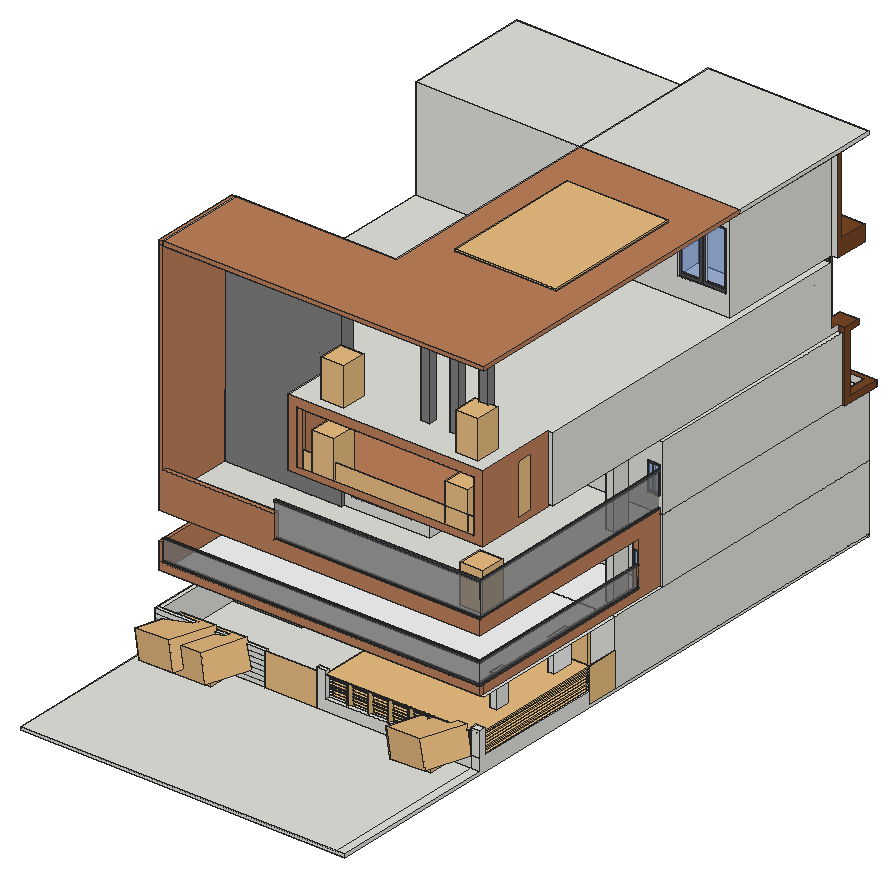
# SketchUp Ruby script. Lengths in inches.
U = 1.inch
M = Sketchup.active_model
def pt(a) = Geom::Point3d.new(a.map { |v| v * U })
def face(e, loops, mat)
  f = e.add_face(loops[0].map { |a| pt(a) })
  loops[1..].each { |l| e.add_face(l.map { |a| pt(a) }).erase! }
  f.material = f.back_material = mat if mat
  f
end
# faces: each face lists its corners as indices into pts; further lists are holes
def faces(e, pts, list, mat = nil) = list.each { |f| face(e, (f[0].is_a?(Array) ? f : [f]).map { |l| l.map { |i| pts[i] } }, mat) }
# xy, xz, yz: faces in a plane at the given z, y or x. An outline is a flat list of corners, or four numbers for a rectangle; further outlines are holes
def ring(l) = l.size == 4 ? [[l[0], l[1]], [l[2], l[1]], [l[2], l[3]], [l[0], l[3]]] : l.each_slice(2).to_a
def flat(e, list, mat, &to3) = list.each { |f| face(e, (f[0].is_a?(Array) ? f : [f]).map { |l| ring(l).map { |u, v| to3.(u, v) } }, mat) }
def xy(e, z, list, mat = nil) = flat(e, list, mat) { |x, y| [x, y, z] }
def xz(e, y, list, mat = nil) = flat(e, list, mat) { |x, z| [x, y, z] }
def yz(e, x, list, mat = nil) = flat(e, list, mat) { |y, z| [x, y, z] }
def lines(e, pts, list) = list.each { |a, b| e.add_line(pt(pts[a]), pt(pts[b])) }
# prism: a flat outline (further loops are holes) pulled along v
def prism(e, loops, v, mat = nil)
  f = face(e, loops, mat); d = Geom::Vector3d.new(v.map { |x| x * U })
  f.pushpull(f.normal.samedirection?(d) ? d.length : -d.length)
end
def box(e, o, s, mat = nil) = prism(e, [[o, [o[0] + s[0], o[1], o[2]], [o[0] + s[0], o[1] + s[1], o[2]], [o[0], o[1] + s[1], o[2]]]], [0, 0, s[2]], mat)
def at(x, y, z, deg = 0) = Geom::Transformation.translation(pt([x, y, z])) * Geom::Transformation.rotation(ORIGIN, Z_AXIS, deg.degrees)
def axes(o, x, y, z) = Geom::Transformation.new([*x, 0, *y, 0, *z, 0, *pt(o).to_a, 1])
def part(name) = M.definitions.add(name)
# library, detail: a bought-in or finely detailed component or shape, given as its bounding box
def library(name, o, s) = part(name).tap { |d| box(d.entities, o, s) }
def detail(e, o, s) = box(e.add_group.entities, o, s)
def put(e, d, t, mat = nil) = e.add_instance(d, t).tap { |i| i.material = mat if mat }
def group(e, t, mat = nil) = e.add_group.tap { |g| g.transformation = t; g.material = mat if mat }.entities
root = M.entities
M.materials.add("GATE RAILINGS").color = [40, 40, 40]
M.materials.add("Material__1").color = [190, 136, 85]
M.materials.add("Material__2").color = [51, 42, 44]
M.materials.add("Material__3").color = [119, 136, 107]
M.materials.add("[0129_WhiteSmoke]").color = [245, 245, 245]
M.materials.add("[0133_Gray]").color = [128, 128, 128]
M.materials.add("[0134_DimGray]").color = [105, 105, 105]
M.materials.add("[0135_DarkGray]").color = [81, 81, 81]
M.materials.add("[Aluminum]1").color = [79, 79, 79]
M.materials.add("[Color_000]").color = [255, 255, 255]
M.materials.add("[Translucent Glass Blue]").color = [100, 149, 237]
M.materials["[Translucent Glass Blue]"].alpha = 0.5
M.materials.add("[Translucent Glass Gray]").color = [128, 128, 128]
M.materials["[Translucent Glass Gray]"].alpha = 0.5
M.materials.add("[Wood Veneer 01]1").color = [120, 70, 37]
M.materials.add("[Wood Veneer 02]").color = [190, 128, 91]
c1 = library("jali15",[0,0,0],[42.92,2.71,85.83])
c2 = library("e203.dxf",[0,0,0],[1.18,1.18,0.01])
c3 = part("Janela aluminio")
xy(c3.entities,0,[[0,0,47.24,1.57],[23.62,1.57,47.24,2.76],[0,2.76,25.98,3.9375],[0,3.9375,47.24,5.91]])
xy(c3.entities,43.31,[[0,0,47.24,1.57],[23.62,1.57,47.24,2.76],[0,2.76,0,5.91,47.24,5.91,47.24,3.9375,25.98,3.9375,25.98,2.76],[25.98,2.76,47.24,3.9375]])
xz(c3.entities,1.57,[[0,0,23.62,0,23.62,41.34,21.26,41.34,21.26,1.97,1.97,1.97,1.97,41.34,23.62,41.34,23.62,43.31,0,43.31],[[23.62,0,47.24,43.31],[25.7,1.97,45.28,41.34]]],"[0135_DarkGray]")
xz(c3.entities,2.76,[[[0,0,23.62,43.31],[2.36,2.36,21.26,40.94]],[23.62,0,25.98,43.31]],"[0135_DarkGray]")
xz(c3.entities,2.76,[[2.36,2.36,21.26,40.94]],"[Translucent Glass Blue]")
xz(c3.entities,3.9375,[[25.98,0,25.98,2.36,44.88,2.36,44.88,40.94,25.98,40.94,25.98,43.31,47.24,43.31,47.24,0]],"[0135_DarkGray]")
xz(c3.entities,3.9375,[[25.98,2.36,44.88,40.94]],"[Translucent Glass Blue]")
yz(c3.entities,0,[[0,0,1.57,43.31],[2.76,0,5.91,43.31]])
yz(c3.entities,23.62,[[1.57,0,2.76,43.31]])
yz(c3.entities,25.98,[[2.76,0,3.9375,43.31]])
yz(c3.entities,47.24,[[0,0,1.57,43.31],[1.57,0,2.76,43.31],[3.9375,0,5.91,43.31]])
c4 = part("bod vindu")
g1 = group(c4.entities,at(0,-46.85,0),"[Translucent Glass Blue]")
yz(g1,0.94,[[2.36,2.36,44.49,19.65]],"[Translucent Glass Blue]")
p = [[0.55,44.49,2.36],[0.94,44.49,2.36],[0.55,2.36,19.65],[0.94,2.36,19.65]]
lines(g1,p,[[0,1],[2,3]])
g2 = group(g1,at(0,46.85,0,-90),"[Color_000]")
xy(g2,0,[[0,0,46.85,3.9375]],"[0135_DarkGray]")
xy(g2,1.57,[[1.57,0,45.28,0.55]],"[0135_DarkGray]")
xy(g2,2.36,[[2.36,0.55,44.49,3.9375]],"[0135_DarkGray]")
xy(g2,19.65,[[2.36,0.55,4.29,3.9375],[4.29,0.55,44.49,3.9375]],"[0135_DarkGray]")
xy(g2,20.43,[[1.57,0,45.28,0.55]],"[0135_DarkGray]")
xy(g2,22.01,[[0,0,46.85,3.9375]],"[0135_DarkGray]")
xz(g2,0,[[[0,0,46.85,22.01],[1.57,1.57,45.28,20.43]]],"[0135_DarkGray]")
xz(g2,0.55,[[1.57,1.57,45.28,2.36],[1.57,2.36,2.36,2.36,2.36,19.65,44.49,19.65,44.49,2.36,45.28,2.36,45.28,20.43,1.57,20.43]],"[0135_DarkGray]")
xz(g2,3.9375,[[[0,0,46.85,22.01],[2.36,2.36,44.49,19.65]]],"[0135_DarkGray]")
yz(g2,0,[[0,0,3.9375,22.01]],"[0135_DarkGray]")
yz(g2,1.57,[[0,1.57,0.55,2.36,0.55,20.43,0,20.43]],"[0135_DarkGray]")
yz(g2,2.36,[[0.55,2.36,3.9375,19.65]],"[0135_DarkGray]")
yz(g2,44.49,[[0.55,2.36,3.9375,19.65]],"[0135_DarkGray]")
yz(g2,45.28,[[0,1.57,0,20.43,0.55,20.43,0.55,2.36]],"[0135_DarkGray]")
yz(g2,46.85,[[0,0,3.9375,22.01]],"[0135_DarkGray]")
p = [[45.28,0,1.57],[1.57,0,1.57],[1.57,0.55,2.36],[2.36,0.55,2.36],[44.49,0.55,2.36],[45.28,0.55,2.36]]
faces(g2,p,[[0,1,2,3,4,5]],"[0135_DarkGray]")
c5 = part("glassesrail")
p = [[933.04,699.08,19.69],[933.04,702.23,19.69]]
lines(c5.entities,p,[[0,1]])
g3 = group(c5.entities,at(14.48,46.28,19.69))
xz(g3,0,[[0.02,0,187.07,0.79,187.06,2.76,0.01,1.97],[0.01,33.46,187.06,34.25,187.05,36.22,0,35.43]],"[Aluminum]1")
xz(g3,1.97,[[0.8,0,0.8,1.97,187.06,2.76,187.07,0.79],[1.98,33.47,1.97,35.44,187.05,36.22,187.06,34.25]],"[Aluminum]1")
p = [[0.8,1.97,0],[0.8,249.26,0],[0.02,249.26,0],[0.02,0,0],[187.07,0,0.79],[187.07,1.97,0.79],
  [0.01,0,1.97],[0.01,249.26,1.97],[0.8,1.97,1.97],[0.8,249.26,1.97],[187.06,0,2.76],[187.06,1.97,2.76],
  [0.01,249.26,33.46],[0.66,249.26,33.47],[1.06,249.26,33.47],[1.98,249.26,33.47],[1.98,1.97,33.47],[187.06,1.97,34.25],
  [187.06,0,34.25],[0.01,0,33.46],[0,0,35.43],[0,249.26,35.43],[1.97,249.26,35.44],[1.97,1.97,35.44],
  [187.05,0,36.22],[187.05,1.97,36.22]]
faces(g3,p,[[0,1,2,3,4,5],[6,7,2,3],[8,9,7,6,10,11],[12,13,14,15,16,17,18,19],[20,21,12,19],[16,15,22,23],[23,22,21,20,24,25]],"[Aluminum]1")
g4 = group(g3,at(0.8,411.86,1.97))
prism(g4,[[[0,-411.07,0],[0,-162.6,0],[0.39,-162.6,0],[0.39,-410.68,0],[185.47,-410.68,0.78],[185.47,-411.07,0.78]]],[-0.13,0,31.5],"[Translucent Glass Gray]")
c6 = library("Glass Railings(black Handrails)",[-57.04,-132.55,0],[169.29,2.52,28.17])
c7 = library("3+80",[0,-4.72,-0.01],[36.22,7.09,85.04])
c8 = library("Porton casa",[13.02,-50.57,0],[86.62,1.75,86.61])
c9 = library("Horizontal railing bar",[-171.26,0.98,-0.71],[237.2,23.72,0.71])
c10 = library("Railing post",[0,-1.77,-6.85],[2.07,1.28,39.37])
c11 = library("Group\#90",[-171.26,0,0],[238.19,24.7,1.97])
c12 = part("Balcony railing")
put(c12.entities,c9,at(44.24,-0.6875,35.43),"GATE RAILINGS")
put(c12.entities,c9,at(44.24,-0.6875,30.79),"GATE RAILINGS")
put(c12.entities,c9,at(44.24,-0.6875,26.14),"GATE RAILINGS")
put(c12.entities,c9,at(44.24,-0.6875,21.5),"GATE RAILINGS")
put(c12.entities,c9,at(44.24,-0.6875,16.85),"GATE RAILINGS")
put(c12.entities,c9,at(44.24,-0.6875,12.2),"GATE RAILINGS")
put(c12.entities,c9,at(44.24,-0.6875,7.56),"GATE RAILINGS")
put(c12.entities,c10,at(60.92,1.38,6.85))
put(c12.entities,c10,at(92.41,1.38,6.85))
put(c12.entities,c10,at(29.42,1.38,6.85))
put(c12.entities,c10,at(-2.07,1.38,6.85))
put(c12.entities,c10,at(-33.57,1.38,6.85))
put(c12.entities,c10,at(-65.07,1.38,6.85))
put(c12.entities,c10,at(-96.5625,1.38,6.85))
put(c12.entities,c11,at(44.24,-0.6875,39.37),"GATE RAILINGS")
c13 = library("Modern Gate 1",[0,0,0],[118.11,1.97,78.74])
c14 = library("cay+chuoi",[26.89,19.66,0.52],[41.96,45.65,69.71])
c15 = library("\#2",[-119.83,-119.83,113.8],[239.66,239.66,17.4])
c16 = library("\#4",[-204.92,-212.35,-236.71],[424.28,257.5,472.53])
c17 = part("\#3")
put(c17.entities,c16,axes([-0.37,309.72,0],[1.36765,0,0],[0,1.36765,0],[0,0,1.36765]),"Material__3")
c18 = library("\#1",[-174.07,-174.07,0],[348.14,348.14,140])
c19 = part("9")
put(c19.entities,c15,at(-19.94,-24.66,0),"Material__2")
put(c19.entities,c17,axes([17.67,-32.6,40.29],[0.29694,0.9549,0],[-0.21403,0.06656,0.97456],[0.9306,-0.28939,0.22414]))
put(c19.entities,c18,at(-19.94,-24.66,0),"Material__1")
xy(root,-6,[[0,0,600,1207],[0,1207,600,1207.75]])
xy(root,0,[[0,0,583.5,310.875],[583.5,0,600,310.875],[203.51,310.875,298.89,317.875],[8,317.875,583.5,317.875,583.5,566.56,600,566.56,600,621.75,324.89,621.75,324.89,484.6875,135.89,484.6875,135.89,480.875,8,480.875],[0,480.875,135.89,480.875,135.89,484.6875,324.89,484.6875,324.89,621.75,600,621.75,600,1207,0,1207],
  [0,1207,600,1207.75]])
xy(root,7.16,[[318.64,517.94,324.89,595.69]])
xy(root,9.32,[[152.3125,484.6875,291.25,502.875]])
xy(root,21.25,[[316.34,310.875,583.5,317.875],[583.5,323.28,600,566.56]])
xy(root,60,[[0,310.875,203.51,317.875],[0,317.875,8,480.875]])
xy(root,67.0625,[[298.89,310.875,316.34,317.875],[583.5,310.875,600,323.28]])
xy(root,101.2,[[152.3125,484.6875,291.25,502.875]])
xy(root,102.03,[[318.64,517.94,324.89,595.69]])
xy(root,120,[[594.25,319,600,621.75],[0,327,8,480.875],[0,480.875,8,488.375],[0,488.375,0,1207.75,600,1207.75,600,732.75,381.34,732.75,381.34,621.75,324.89,621.75,324.89,495.125,165.85,495.125,165.85,488.375],[324.89,495.125,381.34,621.75],
  [561.82,515.52,572.89,555.2],[583.49,621.75,594.25,732.75],[594.25,621.75,600,732.75],[562.02,648.71,577.08,680.89]])
xy(root,120,[[0,319,594.25,327],[[8,327,8,480.875,135.89,480.875,135.89,484.6875,324.89,484.6875,324.89,495.125,381.34,495.125,381.34,621.75,583.49,621.75,583.49,327],[561.82,515.52,572.89,555.2]],[[583.49,327,594.25,621.75],[561.82,381.16,574.2,408.78]],[8,480.875,8,488.375,165.85,488.375,165.85,495.125,324.89,495.125,324.89,484.6875,135.89,484.6875,135.89,480.875],[[381.34,621.75,583.49,732.75],[562.02,648.71,577.08,680.89]]],"[0129_WhiteSmoke]")
xy(root,127.77,[[362.03,644.59,381.34,705.65]])
xy(root,132.96,[[177.95,495.125,345.45,525.4375]])
xy(root,134.375,[[0,319,8,327]])
xy(root,134.375,[[8,319,594.25,327],[583.49,327,594.25,684.5625]],"[Wood Veneer 02]")
xy(root,168,[[0,319,8,488.375]],"[Wood Veneer 02]")
xy(root,172.76,[[585.65,684.5625,592.33,691]])
xy(root,199.19,[[585.65,684.5625,592.33,691]])
xy(root,200.65,[[362.03,644.59,381.34,705.65]])
xy(root,206.77,[[177.95,495.125,345.45,525.4375]])
xy(root,218.53,[[0,319,0,488.375,31.26,488.375,31.26,354.9375,583.49,354.9375,583.49,684.5625,594.25,684.5625,594.25,319],[31.26,354.9375,31.26,488.375,165.85,488.375,165.85,495.125,381.34,495.125,381.34,732.75,583.49,732.75,583.49,354.9375]],"[Wood Veneer 02]")
xy(root,240,[[8,327,586.25,327,586.25,732.75,381.34,732.75,381.34,468.0625,223.57,468.0625,223.57,462,8,462],[8,462,8,488.375,0,488.375,0,1145.375,600,1145.375,600,732.75,381.34,732.75,381.34,468.0625,223.57,468.0625,223.57,462],[[0,1145.375,591.125,1207.75],[535.76,1182.9375,537.8,1183.37,539.66,1184.32,541.22,1185.72,542.36,1187.47,543,1189.45,543.11,1191.54,542.68,1193.58,541.73,1195.44,540.33,1197,538.58,1198.13,536.6,1198.78,534.51,1198.89,532.47,1198.46,530.61,1197.51,529.06,1196.11,527.92,1194.36,527.27,1192.375,527.16,1190.29,527.59,1188.25,528.54,1186.39,529.9375,1184.83,531.6875,1183.7,533.67,1183.05]],[591.125,1145.375,600,1207.75],[600,1145.375,606.25,1218.25],
  [535.76,1182.9375,533.67,1183.05,531.6875,1183.7,529.9375,1184.83,528.54,1186.39,527.59,1188.25,527.16,1190.29,527.27,1192.375,527.92,1194.36,529.06,1196.11,530.61,1197.51,532.47,1198.46,534.51,1198.89,536.6,1198.78,538.58,1198.13,540.33,1197,541.73,1195.44,542.68,1193.58,543.11,1191.54,543,1189.45,542.36,1187.47,541.22,1185.72,539.66,1184.32,537.8,1183.37],[0,1207.75,600,1218.25]])
xy(root,245.125,[[214.63,319,594.25,319,594.25,732.75,586.25,732.75,586.25,327,214.63,327]],"[Wood Veneer 02]")
xy(root,252.33,[[591.125,1157.8125,606.25,1157.8125,606.25,1218.25,0,1218.25,0,1207.75,591.125,1207.75]],"[Wood Veneer 01]1")
xy(root,257.15,[[366.9,548.34,381.34,682.41]])
xy(root,258.5625,[[238.35,468.0625,348.91,499.75]])
xy(root,269.16,[[572.59,732.75,593.96,740.9375]])
xy(root,288,[[8,319,214.63,327]],"[Wood Veneer 02]")
xy(root,321.6,[[572.59,732.75,593.96,740.9375]])
xy(root,332.02,[[366.9,548.34,381.34,682.41]])
xy(root,335,[[238.35,468.0625,348.91,499.75]])
xy(root,354.5625,[[223.57,468.0625,381.34,487.75]])
xy(root,354.5625,[[223.57,337.625,223.57,468.0625,381.34,468.0625,381.34,487.75,584.16,487.75,584.16,337.625]],"[Wood Veneer 02]")
xy(root,360,[[0,462,8,488.375],[[381.34,487.75,592.625,732.75],[562.02,648.71,577.08,680.89]],[592.625,732.75,600,1145.375],[0,1091.625,584.625,1145.375],[584.625,1091.625,592.625,1145.375]])
xy(root,360,[[571.27,1145.375,571.27,1177.4375,606.25,1177.4375,606.25,1157.8125,591.125,1157.8125,591.125,1145.375]],"[Wood Veneer 01]1")
xy(root,366,[[240.32,337.625,251.32,341.6875]])
xy(root,366,[[251.32,337.625,567.35,337.625,567.35,487.75,240.32,487.75,240.32,341.6875,251.32,341.6875]],"[Wood Veneer 02]")
xy(root,368.23,[[581.85,419.93,584.16,446.93]])
xy(root,370.12,[[578.4375,1091.625,584.625,1130]])
xy(root,370.12,[[0,1091.625,578.4375,1091.625,578.4375,1130,592.625,1130,592.625,1145.375,606.25,1145.375,606.25,1177.4375,571.27,1177.4375,571.27,1145.375,0,1145.375]],"[Wood Veneer 01]1")
xy(root,372.74,[[290.9,487.75,461.27,551.125]])
xy(root,455.86,[[290.9,487.75,461.27,551.125]])
xy(root,458.42,[[581.85,419.93,584.16,446.93]],"[Wood Veneer 02]")
xy(root,464.6875,[[251.32,337.625,251.32,341.6875,240.32,341.6875,240.32,487.75,567.35,487.75,567.35,337.625]],"[Wood Veneer 02]")
xy(root,480,[[[223.57,337.625,584.16,337.625,584.16,487.75,592.625,487.75,592.625,1130,580.6875,1130,580.6875,911.92,0,911.92,0,487.75,223.57,487.75],[420.56,398.17,437.44,411.49],[474.66,398.17,491.53,411.49],[528.75,398.17,545.63,411.49]],[[0,1091.625,0,1207.75,592.625,1207.75,592.625,1145.375,578.4375,1145.375,578.4375,1091.625],[535.76,1182.9375,537.8,1183.37,539.66,1184.32,541.22,1185.72,542.36,1187.47,543,1189.45,543.11,1191.54,542.68,1193.58,541.73,1195.44,540.33,1197,538.58,1198.13,536.6,1198.78,534.51,1198.89,532.47,1198.46,530.61,1197.51,529.06,1196.11,527.92,1194.36,527.27,1192.375,527.16,1190.29,527.59,1188.25,528.54,1186.39,529.9375,1184.83,531.6875,1183.7,533.67,1183.05]],[578.4375,1130,580.6875,1145.375]])
xy(root,509.8125,[[0,1145.375,573,1145.375,573,1153.6875,592.625,1153.6875,592.625,1207.75,0,1207.75]],"[Wood Veneer 01]1")
xy(root,516.3125,[[484.875,911.92,572.5,958.23]])
xy(root,625.25,[[484.875,911.92,572.5,958.23]])
xy(root,651.0625,[[528.75,398.17,545.63,411.49]])
xy(root,658.8125,[[0,319,8,462],[8,462,223.57,487.75],[580.6875,911.92,600,1145.375],[304,1145.375,573,1207.75],[592.625,1145.375,600,1207.75],
  [573,1153.6875,592.625,1207.75]])
xy(root,658.8125,[[[8,319,8,462,223.57,462,223.57,487.75,304,487.75,304,1145.375,580.6875,1145.375,580.6875,911.92,600,911.92,600,319],[355.23,559.36,541.86,818.43],[420.56,398.17,437.44,411.49],[474.66,398.17,491.53,411.49]]],"[Wood Veneer 02]")
xy(root,665.9375,[[0,911.92,304,1145.375],[304,911.92,600,1207.75]])
xy(root,665.9375,[[0,319,8,488.375],[[8,319,600,319,600,911.92,304,911.92,304,487.75,8,487.75],[355.23,559.36,541.86,818.43]]],"[Wood Veneer 02]")
xz(root,0,[[0,-6,600,0]])
xz(root,310.875,[[0,0,203.51,60],[298.89,0,583.5,0,583.5,21.25,316.34,21.25,316.34,67.0625,298.89,67.0625],[583.5,0,600,21.25],[583.5,21.25,600,67.0625]])
xz(root,317.875,[[8,0,203.51,60],[298.89,0,298.89,67.0625,316.34,67.0625,316.34,21.25,583.5,21.25,583.5,0]])
xz(root,319,[[0,120,594.25,134.375],[0,134.375,8,168],[0,218.53,594.25,218.53,594.25,245.125,214.63,245.125,214.63,288,8,288,8,658.8125,0,658.8125],[0,658.8125,8,665.9375],[8,658.8125,600,665.9375]],"[Wood Veneer 02]")
xz(root,323.28,[[583.5,21.25,600,67.0625]])
xz(root,327,[[0,120,8,134.375],[583.49,120,594.25,134.375]])
xz(root,327,[[8,120,583.49,134.375],[8,240,214.63,288],[214.63,240,586.25,245.125]],"[Wood Veneer 02]")
xz(root,337.625,[[[223.57,354.5625,584.16,480],[240.32,366,567.35,464.6875]],[240.32,366,251.32,464.6875]],"[Wood Veneer 02]")
xz(root,341.6875,[[240.32,366,251.32,464.6875]])
xz(root,354.9375,[[31.26,218.53,583.49,232]])
xz(root,381.16,[[561.82,0,574.2,120]])
xz(root,398.17,[[420.56,480,437.44,658.8125],[474.66,480,491.53,658.8125],[528.75,480,545.63,651.0625]],"[0133_Gray]")
xz(root,408.78,[[561.82,0,574.2,120]])
xz(root,411.49,[[420.56,480,437.44,658.8125],[474.66,480,491.53,658.8125],[528.75,480,545.63,651.0625]],"[0133_Gray]")
xz(root,419.93,[[581.85,368.23,584.16,458.42]],"[Wood Veneer 02]")
xz(root,446.93,[[581.85,368.23,584.16,458.42]],"[Wood Veneer 02]")
xz(root,462,[[8,240,223.57,240,223.57,658.8125,0,658.8125,0,360,8,360]],"[0133_Gray]")
xz(root,468.0625,[[[223.57,240,381.34,354.5625],[238.35,258.5625,348.91,335]]])
xz(root,480.875,[[0,0,8,60]])
xz(root,480.875,[[8,0,135.89,0,135.89,120,0,120,0,60,8,60]],"[0133_Gray]")
xz(root,484.6875,[[[135.89,0,324.89,120],[152.3125,9.32,291.25,101.2]]])
xz(root,487.75,[[223.57,354.5625,381.34,360],[381.34,354.5625,584.16,360],[584.16,360,592.625,480],[[240.32,366,567.35,464.6875],[290.9,372.74,461.27,455.86]]])
xz(root,487.75,[[8,658.8125,304,665.9375]],"[Wood Veneer 02]")
xz(root,488.375,[[0,120,8,168],[0,240,8,360]])
xz(root,488.375,[[8,120,165.85,120,165.85,218.53,0,218.53,0,168,8,168]],"[0133_Gray]")
xz(root,488.375,[[0,360,8,665.9375]],"[Wood Veneer 02]")
xz(root,495.125,[[[165.85,120,381.34,218.53],[177.95,132.96,345.45,206.77]]])
xz(root,499.75,[[238.35,258.5625,348.91,335]])
xz(root,502.875,[[152.3125,9.32,291.25,101.2]])
xz(root,515.52,[[561.82,0,572.89,120]])
xz(root,517.94,[[318.64,7.16,324.89,102.03]])
xz(root,525.4375,[[177.95,132.96,345.45,206.77]])
xz(root,548.34,[[366.9,257.15,381.34,332.02]])
xz(root,551.125,[[290.9,372.74,461.27,455.86]])
xz(root,555.2,[[561.82,0,572.89,120]],"[0129_WhiteSmoke]")
xz(root,559.36,[[355.23,658.8125,541.86,665.9375]],"[Wood Veneer 02]")
xz(root,566.56,[[583.5,0,600,21.25]])
xz(root,595.69,[[318.64,7.16,324.89,102.03]])
xz(root,621.75,[[324.89,0,600,120]])
xz(root,644.59,[[362.03,127.77,381.34,200.65]])
xz(root,648.71,[[562.02,120,577.08,360]])
xz(root,680.89,[[562.02,120,577.08,360]])
xz(root,682.41,[[366.9,257.15,381.34,332.02]])
xz(root,684.5625,[[[583.49,134.375,594.25,218.53],[585.65,172.76,592.33,199.19]]],"[Wood Veneer 02]")
xz(root,691,[[585.65,172.76,592.33,199.19]])
xz(root,705.65,[[362.03,127.77,381.34,200.65]])
xz(root,732.75,[[381.34,120,583.49,218.53],[583.49,120,594.25,232],[594.25,120,600,240],[[381.34,240,586.25,240,586.25,245.125,594.25,245.125,594.25,240,600,240,600,360,381.34,360],[572.59,269.16,593.96,321.6]],[586.25,240,594.25,245.125]])
xz(root,740.9375,[[572.59,269.16,593.96,321.6]])
xz(root,818.43,[[355.23,658.8125,541.86,665.9375]],"[Wood Veneer 02]")
xz(root,911.92,[[[0,480,580.6875,480,580.6875,658.8125,600,658.8125,600,665.9375,0,665.9375],[484.875,516.3125,572.5,625.25]]])
xz(root,958.23,[[484.875,516.3125,572.5,625.25]])
xz(root,1091.625,[[0,370.12,578.4375,480]])
xz(root,1130,[[578.4375,370.12,592.625,480]],"[Wood Veneer 01]1")
xz(root,1145.375,[[0,240,591.125,360],[591.125,240,592.625,360],[592.625,240,600,360],[580.6875,480,592.625,658.8125],[0,509.8125,0,665.9375,304,665.9375,304,658.8125,573,658.8125,573,509.8125]])
xz(root,1145.375,[[600,240,606.25,360],[0,360,571.27,370.12],[592.625,360,606.25,370.12]],"[Wood Veneer 01]1")
xz(root,1153.6875,[[573,509.8125,592.625,658.8125]],"[Wood Veneer 01]1")
xz(root,1157.8125,[[591.125,252.33,606.25,360]],"[Wood Veneer 01]1")
xz(root,1177.4375,[[571.27,360,606.25,370.12]],"[Wood Veneer 01]1")
xz(root,1207,[[0,-6,600,0]])
xz(root,1207.75,[[0,0,600,120],[0,120,600,240],[0,240,591.125,252.33],[304,658.8125,600,665.9375]])
xz(root,1207.75,[[0,480,592.625,509.8125]],"[Wood Veneer 01]1")
xz(root,1218.25,[[0,240,606.25,252.33]],"[Wood Veneer 01]1")
yz(root,0,[[0,-6,0,0,310.875,0,310.875,60,480.875,60,480.875,0,1207,0,1207,-6],[1207,-6,1207.75,0],[480.875,0,1207.75,120],[319,120,327,134.375],[488.375,120,488.375,232,319,232,319,658.8125,462,658.8125,462,360,488.375,360,488.375,240,1207.75,240,1207.75,120],
  [319,218.53,488.375,232],[488.375,240,1145.375,360],[462,360,462,658.8125,319,658.8125,319,665.9375,487.75,665.9375,487.75,480,488.375,480,488.375,360],[488.375,360,488.375,480,911.92,480,911.92,665.9375,1145.375,665.9375,1145.375,480,1091.625,480,1091.625,360],[487.75,480,488.375,665.9375]])
yz(root,0,[[1207.75,240,1218.25,252.33],[1091.625,360,1145.375,370.12],[1145.375,480,1207.75,509.8125]],"[Wood Veneer 01]1")
yz(root,0,[[327,120,327,134.375,319,134.375,319,168,488.375,168,488.375,120]],"[Wood Veneer 02]")
yz(root,8,[[317.875,0,480.875,60],[462,240,488.375,360],[319,658.8125,487.75,665.9375]])
yz(root,8,[[327,120,488.375,120,488.375,168,319,168,319,134.375,327,134.375],[327,240,462,240,462,360,488.375,360,488.375,665.9375,487.75,665.9375,487.75,658.8125,319,658.8125,319,288,327,288]],"[Wood Veneer 02]")
yz(root,31.26,[[354.9375,218.53,488.375,232]])
yz(root,135.89,[[480.875,0,484.6875,120]],"[0133_Gray]")
yz(root,152.3125,[[484.6875,9.32,502.875,101.2]])
yz(root,165.85,[[488.375,120,495.125,218.53]],"[0133_Gray]")
yz(root,177.95,[[495.125,132.96,525.4375,206.77]])
yz(root,203.51,[[310.875,0,317.875,60]])
yz(root,214.63,[[319,245.125,327,288]],"[Wood Veneer 02]")
yz(root,223.57,[[337.625,354.5625,462,480],[462,354.5625,487.75,360],[462,360,487.75,480]])
yz(root,223.57,[[462,240,468.0625,354.5625],[462,480,487.75,658.8125]],"[0133_Gray]")
yz(root,238.35,[[468.0625,258.5625,499.75,335]])
yz(root,240.32,[[337.625,366,341.6875,464.6875]])
yz(root,240.32,[[341.6875,366,487.75,464.6875]],"[Wood Veneer 02]")
yz(root,251.32,[[337.625,366,341.6875,464.6875]],"[Wood Veneer 02]")
yz(root,290.9,[[487.75,372.74,551.125,455.86]])
yz(root,291.25,[[484.6875,9.32,502.875,101.2]])
yz(root,298.89,[[310.875,0,317.875,67.0625]])
yz(root,304,[[487.75,658.8125,1145.375,665.9375],[1145.375,658.8125,1207.75,665.9375]])
yz(root,316.34,[[310.875,21.25,317.875,67.0625]])
yz(root,318.64,[[517.94,7.16,595.69,102.03]])
yz(root,324.89,[[[484.6875,0,621.75,120],[517.94,7.16,595.69,102.03]]])
yz(root,345.45,[[495.125,132.96,525.4375,206.77]])
yz(root,348.91,[[468.0625,258.5625,499.75,335]])
yz(root,355.23,[[559.36,658.8125,818.43,665.9375]],"[Wood Veneer 02]")
yz(root,362.03,[[644.59,127.77,705.65,200.65]])
yz(root,366.9,[[548.34,257.15,682.41,332.02]])
yz(root,381.34,[[[495.125,120,732.75,218.53],[644.59,127.77,705.65,200.65]],[[468.0625,240,732.75,240,732.75,360,487.75,360,487.75,354.5625,468.0625,354.5625],[548.34,257.15,682.41,332.02]]])
yz(root,420.56,[[398.17,480,411.49,658.8125]],"[0133_Gray]")
yz(root,437.44,[[398.17,480,411.49,658.8125]],"[0133_Gray]")
yz(root,461.27,[[487.75,372.74,551.125,455.86]])
yz(root,474.66,[[398.17,480,411.49,658.8125]],"[0133_Gray]")
yz(root,484.875,[[911.92,516.3125,958.23,625.25]])
yz(root,491.53,[[398.17,480,411.49,658.8125]],"[0133_Gray]")
yz(root,528.75,[[398.17,480,411.49,651.0625]],"[0133_Gray]")
yz(root,541.86,[[559.36,658.8125,818.43,665.9375]],"[Wood Veneer 02]")
yz(root,545.63,[[398.17,480,411.49,651.0625]],"[0133_Gray]")
yz(root,561.82,[[381.16,0,408.78,120]])
yz(root,561.82,[[515.52,0,555.2,120]],"[0129_WhiteSmoke]")
yz(root,562.02,[[648.71,120,680.89,360]])
yz(root,567.35,[[337.625,366,487.75,464.6875]],"[Wood Veneer 02]")
yz(root,571.27,[[1145.375,360,1177.4375,370.12]],"[Wood Veneer 01]1")
yz(root,572.5,[[911.92,516.3125,958.23,625.25]])
yz(root,572.59,[[732.75,269.16,740.9375,321.6]])
yz(root,572.89,[[515.52,0,555.2,120]],"[0129_WhiteSmoke]")
yz(root,573,[[1145.375,509.8125,1153.6875,658.8125]],"[Wood Veneer 01]1")
yz(root,574.2,[[381.16,0,408.78,120]])
yz(root,577.08,[[648.71,120,680.89,360]])
yz(root,578.4375,[[1091.625,458.4375,1130,480]])
yz(root,578.4375,[[1091.625,370.12,1130,458.4375]],"[Wood Veneer 01]1")
yz(root,580.6875,[[911.92,480,1145.375,658.8125]])
yz(root,581.85,[[419.93,368.23,446.93,458.42]],"[Wood Veneer 02]")
yz(root,583.49,[[354.9375,218.53,732.75,232]])
yz(root,583.49,[[327,120,327,134.375,684.5625,134.375,684.5625,218.53,732.75,218.53,732.75,120]],"[Wood Veneer 02]")
yz(root,583.5,[[317.875,0,317.875,21.25,310.875,21.25,310.875,67.0625,323.28,67.0625,323.28,21.25,566.56,21.25,566.56,0]])
yz(root,584.16,[[[337.625,354.5625,487.75,480],[419.93,368.23,446.93,458.42]]],"[Wood Veneer 02]")
yz(root,585.65,[[684.5625,172.76,691,199.19]])
yz(root,586.25,[[327,240,732.75,245.125]])
yz(root,591.125,[[1145.375,240,1145.375,360,1157.8125,360,1157.8125,252.33,1207.75,252.33,1207.75,240]],"[Wood Veneer 01]1")
yz(root,592.33,[[684.5625,172.76,691,199.19]])
yz(root,592.625,[[487.75,360,1145.375,360,1145.375,370.12,1130,370.12,1130,480,487.75,480]])
yz(root,592.625,[[1145.375,480,1207.75,480,1207.75,509.8125,1153.6875,509.8125,1153.6875,658.8125,1145.375,658.8125]],"[Wood Veneer 01]1")
yz(root,593.96,[[732.75,269.16,740.9375,321.6]])
yz(root,594.25,[[319,120,327,134.375],[327,120,732.75,120,732.75,245.125,319,245.125,319,218.53,684.5625,218.53,684.5625,134.375,327,134.375]],"[Wood Veneer 02]")
yz(root,600,[[0,-6,1207,-6,1207,0,566.56,0,566.56,21.25,323.28,21.25,323.28,67.0625,310.875,67.0625,310.875,0,0,0],[1207,-6,1207.75,0],[621.75,0,1207.75,120],[732.75,120,1207.75,240],[732.75,240,1145.375,360],
  [911.92,658.8125,1207.75,665.9375]])
yz(root,600,[[319,658.8125,911.92,665.9375]],"[Wood Veneer 02]")
yz(root,606.25,[[1145.375,240,1218.25,240,1218.25,252.33,1157.8125,252.33,1157.8125,360,1177.4375,360,1177.4375,370.12,1145.375,370.12]],"[Wood Veneer 01]1")
p = [[533.67,1183.05,240],[535.76,1182.9375,240],[535.76,1182.9375,480],[533.67,1183.05,480],[537.8,1183.37,240],[537.8,1183.37,480],
  [531.6875,1183.7,240],[531.6875,1183.7,480],[539.66,1184.32,240],[539.66,1184.32,480],[529.9375,1184.83,240],[529.9375,1184.83,480],
  [541.22,1185.72,240],[541.22,1185.72,480],[528.54,1186.39,240],[528.54,1186.39,480],[542.36,1187.47,240],[542.36,1187.47,480],
  [527.59,1188.25,240],[527.59,1188.25,480],[543,1189.45,240],[543,1189.45,480],[527.16,1190.29,240],[527.16,1190.29,480],
  [543.11,1191.54,240],[543.11,1191.54,480],[527.27,1192.375,240],[527.27,1192.375,480],[542.68,1193.58,240],[542.68,1193.58,480],
  [527.92,1194.36,240],[527.92,1194.36,480],[541.73,1195.44,240],[541.73,1195.44,480],[529.06,1196.11,240],[529.06,1196.11,480],
  [540.33,1197,240],[540.33,1197,480],[530.61,1197.51,240],[530.61,1197.51,480],[538.58,1198.13,240],[538.58,1198.13,480],
  [532.47,1198.46,240],[532.47,1198.46,480],[536.6,1198.78,240],[536.6,1198.78,480],[534.51,1198.89,240],[534.51,1198.89,480],
  [223.57,487.75,658.8125],[223.57,487.75,480],[8,488.375,480],[8,488.375,658.8125],[0,488.375,232],[31.26,488.375,232],
  [183.42,471.28,480],[183.42,462,480],[584.625,1091.625,360],[584.625,1091.625,370.12],[584.625,1091.625,458.4375],[592.625,1091.625,458.4375],
  [584.625,1145.375,360],[584.625,1145.375,370.12],[-0.26,310.875,51.41],[0,310.875,51.41],[203.25,310.875,51.41],[-0.53,310.875,42.83],
  [0,310.875,42.83],[202.98,310.875,42.83],[-0.79,310.875,34.24],[0,310.875,34.24],[202.72,310.875,34.24],[-1.05,310.875,25.65],
  [0,310.875,25.65],[202.46,310.875,25.65],[-1.31,310.875,17.07],[0,310.875,17.07],[202.2,310.875,17.07],[-1.58,310.875,8.48],
  [0,310.875,8.48],[201.93,310.875,8.48],[-1.84,310.875,-0.11],[201.67,310.875,-0.11]]
faces(root,p,[[0,1,2,3],[1,4,5,2],[6,0,3,7],[4,8,9,5],[10,6,7,11],[8,12,13,9],[14,10,11,15],[12,16,17,13],
  [18,14,15,19],[16,20,21,17],[22,18,19,23],[20,24,25,21],[26,22,23,27],[24,28,29,25],[30,26,27,31],[28,32,33,29],
  [34,30,31,35],[32,36,37,33],[38,34,35,39],[36,40,41,37],[42,38,39,43],[40,44,45,41],[46,42,43,47],[44,46,47,45]],"[0134_DimGray]")
faces(root,p,[[48,49,50,51]],"[Wood Veneer 02]")
lines(root,p,[[52,53],[54,55],[56,57],[58,59],[60,61],[62,63],[63,64],[65,66],[66,67],[68,69],[69,70],[71,72],
  [72,73],[74,75],[75,76],[77,78],[78,79],[80,81]])
put(root,c1,axes([584.16,419.93,368.23],[0,0.62914,0],[-1,0,0],[0,0,1.05076]))
put(root,c2,axes([355.23,559.36,658.8125],[158.00917,0,0],[0,219.33958,0],[0,0,1036.36364]))
put(root,c3,axes([238.35,468.0625,258.5625],[2.34024,0,0],[0,1,0],[0,0,1.76501]))
put(root,c3,axes([177.95,495.125,132.96],[3.54542,0,0],[0,1,0],[0,0,1.7044]))
put(root,c3,axes([151.94,484.6875,9.32],[2.9487,0,0],[0,1,0],[0,0,2.12148]))
put(root,c3,axes([381.34,548.625,257.15],[0,2.83169,0],[-1,0,0],[0,0,1.72893]))
put(root,c3,axes([381.34,644.59,127.77],[0,1.29249,0],[-1,0,0],[0,0,1.68275]))
put(root,c3,axes([324.89,517.94,7.16],[0,1.64571,0],[-1,0,0],[0,0,2.19075]))
put(root,c3,axes([290.9,487.75,372.74],[3.60627,0,0],[0,1,0],[0,0,1.91943]))
put(root,c3,axes([573.29,734.33,269.16],[0.43762,0,0],[0,-0.49034,0],[0,0,1.19298]))
put(root,c4,axes([592.33,684.5625,172.76],[0,0.53,0],[0,0,-0.5643],[-0.30387,0,0]))
put(root,c3,axes([484.875,911.92,516.3125],[1.85473,0,0],[0,1.54,0],[0,0,2.54162]))
put(root,c5,axes([703.01,290.61,111.74],[0,1.96,0],[-2.35,0,0],[0,0,1.15]))
put(root,c5,axes([664.94,286.63,205.95],[0,2.2344,0],[-1.5275,0,0],[0,0,1.89]))
put(root,c6,axes([357.8125,470.18,366],[1.86675,0,0],[0,1,0],[0,0,1.12]))
put(root,c7,at(518.06,621.75,0))
put(root,c8,axes([189.17,353.25,-6.61],[1.10125,0,0],[0,0.83785,0],[0,0,0.77026]))
put(root,c12,axes([467.25,317.98,13.81],[1.18811,0,0],[0,10.3141,0],[0,0,1.18]))
put(root,c13,axes([598.03,622.07,0],[0,-0.48602,0],[1.35,0,0],[0,0,0.79419]))
put(root,c14,at(515.31,317.96,243.71))
put(root,c14,at(487.79,318.01,368.48))
put(root,c14,at(241.31,317.21,366.63))
put(root,c14,at(243.28,336.4,479.48))
put(root,c14,at(491.66,336.4,479.48))
put(root,c19,axes([62.5,288.87,1.89],[0.14,0,0],[0,0.14,0],[0,0,0.14]))
put(root,c19,axes([121.4375,288.87,1.89],[0.14,0,0],[0,0.14,0],[0,0,0.14]))
put(root,c19,axes([527.13,288.87,1.89],[0.14,0,0],[0,0.14,0],[0,0,0.14]))
